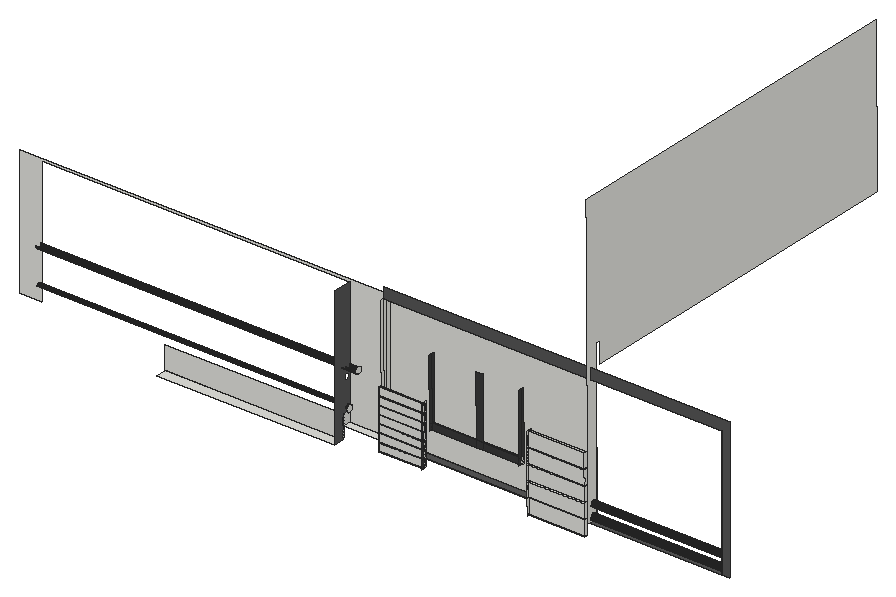
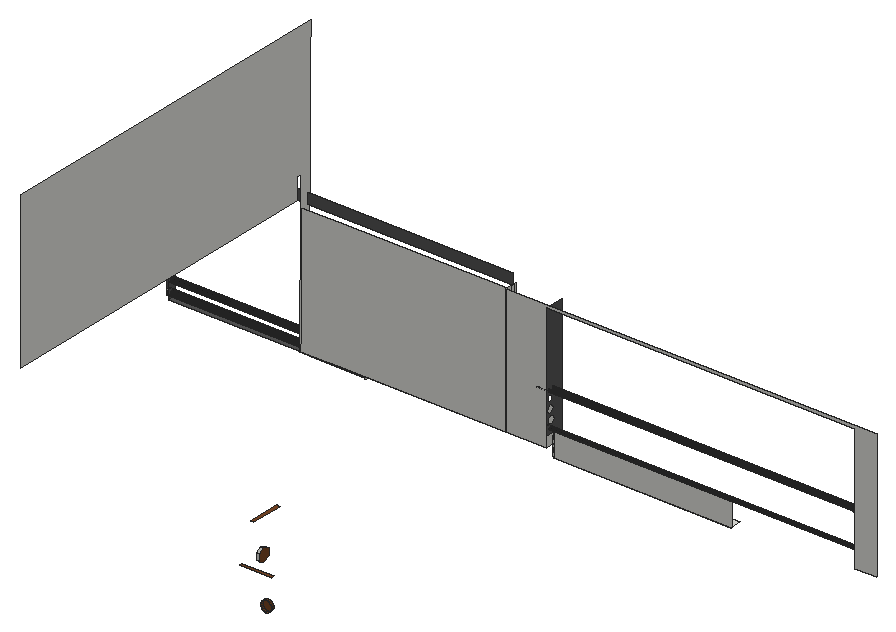
# SketchUp Ruby script. Lengths in inches.
U = 1.inch
M = Sketchup.active_model
def pt(a) = Geom::Point3d.new(a.map { |v| v * U })
def face(e, loops, mat)
  f = e.add_face(loops[0].map { |a| pt(a) })
  loops[1..].each { |l| e.add_face(l.map { |a| pt(a) }).erase! }
  f.material = f.back_material = mat if mat
  f
end
# faces: each face lists its corners as indices into pts; further lists are holes
def faces(e, pts, list, mat = nil) = list.each { |f| face(e, (f[0].is_a?(Array) ? f : [f]).map { |l| l.map { |i| pts[i] } }, mat) }
# xy, xz, yz: faces in a plane at the given z, y or x. An outline is a flat list of corners, or four numbers for a rectangle; further outlines are holes
def ring(l) = l.size == 4 ? [[l[0], l[1]], [l[2], l[1]], [l[2], l[3]], [l[0], l[3]]] : l.each_slice(2).to_a
def flat(e, list, mat, &to3) = list.each { |f| face(e, (f[0].is_a?(Array) ? f : [f]).map { |l| ring(l).map { |u, v| to3.(u, v) } }, mat) }
def xy(e, z, list, mat = nil) = flat(e, list, mat) { |x, y| [x, y, z] }
def xz(e, y, list, mat = nil) = flat(e, list, mat) { |x, z| [x, y, z] }
def yz(e, x, list, mat = nil) = flat(e, list, mat) { |y, z| [x, y, z] }
def lines(e, pts, list) = list.each { |a, b| e.add_line(pt(pts[a]), pt(pts[b])) }
# prism: a flat outline (further loops are holes) pulled along v
def prism(e, loops, v, mat = nil)
  f = face(e, loops, mat); d = Geom::Vector3d.new(v.map { |x| x * U })
  f.pushpull(f.normal.samedirection?(d) ? d.length : -d.length)
end
def box(e, o, s, mat = nil) = prism(e, [[o, [o[0] + s[0], o[1], o[2]], [o[0] + s[0], o[1] + s[1], o[2]], [o[0], o[1] + s[1], o[2]]]], [0, 0, s[2]], mat)
def at(x, y, z, deg = 0) = Geom::Transformation.translation(pt([x, y, z])) * Geom::Transformation.rotation(ORIGIN, Z_AXIS, deg.degrees)
def axes(o, x, y, z) = Geom::Transformation.new([*x, 0, *y, 0, *z, 0, *pt(o).to_a, 1])
def part(name) = M.definitions.add(name)
# library, detail: a bought-in or finely detailed component or shape, given as its bounding box
def library(name, o, s) = part(name).tap { |d| box(d.entities, o, s) }
def detail(e, o, s) = box(e.add_group.entities, o, s)
def put(e, d, t, mat = nil) = e.add_instance(d, t).tap { |i| i.material = mat if mat }
def group(e, t, mat = nil) = e.add_group.tap { |g| g.transformation = t; g.material = mat if mat }.entities
root = M.entities
M.materials.add("[0136_Charcoal]").color = [35, 35, 35]
M.materials.add("[Color M06]").color = [86, 86, 86]
M.materials.add("[Color M07]").color = [58, 58, 58]
M.materials.add("[Wood Veneer 01]").color = [120, 70, 37]
xy(root,214.25,[[350.625,15,549.5625,26.8125]])
xy(root,228,[[549.5625,27,595.0625,36]])
xy(root,228,[[595.0625,27,973.625,36]],"[Color M06]")
xy(root,276,[[614,330.04,617,366.04],[539.92,430.1875,575.92,433.1875]],"[Wood Veneer 01]")
xy(root,286.06,[[762.91,22.06,825.84,22.1875]])
xz(root,26.8125,[[349.93,214.25,549.5625,240]])
xz(root,27,[[595.0625,227.94,784.34,228],[595.0625,227.94,825.84,228],[784.34,227.94,825.84,228]])
xz(root,27,[[973.625,228,982.625,228,982.625,384,595.0625,384,595.0625,372,973.625,372]],"[Color M06]")
xz(root,36,[[180.5,228,180.5,372,595.0625,372,595.0625,228,549.5625,228,549.5625,368.875,204.375,368.875,204.375,228]])
xz(root,348.94,[[611,235.8,614,243.23]],"[Wood Veneer 01]")
xz(root,361.82,[[611,235.8,614,243.23]])
xz(root,427.1875,[[548.71,236.42,550.32,236.63,551.81,237.25,553.09,238.24,554.07,239.52,554.69,241.01,554.9,242.61,554.69,244.21,554.07,245.7,553.09,246.99,551.81,247.97,550.32,248.59,548.71,248.8,547.11,248.59,545.62,247.97,544.34,246.99,543.36,245.7,542.74,244.21,542.53,242.61,542.74,241.01,543.36,239.52,544.34,238.24,545.62,237.25,547.11,236.63]],"[Wood Veneer 01]")
yz(root,548.3125,[[31.79,251.75,32.66,251.86,33.47,252.2,34.17,252.73,34.71,253.43,35.05,254.25,35.16,255.12,35.05,255.99,34.71,256.81,34.17,257.51,33.47,258.04,32.66,258.38,31.79,258.5,30.91,258.38,30.1,258.04,29.4,257.51,28.86,256.81,28.53,255.99,28.41,255.12,28.53,254.25,28.86,253.43,29.4,252.73,30.1,252.2,30.91,251.86]])
yz(root,549.4375,[[31.79,262.25,32.66,262.36,33.47,262.7,34.17,263.23,34.71,263.93,35.05,264.75,35.16,265.62,35.05,266.49,34.71,267.31,34.17,268.01,33.47,268.54,32.66,268.88,31.79,269,30.91,268.88,30.1,268.54,29.4,268.01,28.86,267.31,28.53,266.49,28.41,265.62,28.53,264.75,28.86,263.93,29.4,263.23,30.1,262.7,30.91,262.36]])
yz(root,549.5625,[[26.8125,216.1875,27,228],[26.8125,228,27,240],[27,228,36,240]])
yz(root,549.5625,[[[15,214.25,15,368.875,36,368.875,36,240,26.8125,240,26.8125,214.25],[31.79,272.75,32.66,272.86,33.47,273.2,34.17,273.73,34.71,274.43,35.05,275.25,35.16,276.12,35.05,276.99,34.71,277.81,34.17,278.51,33.47,279.04,32.66,279.38,31.79,279.5,30.91,279.38,30.1,279.04,29.4,278.51,28.86,277.81,28.53,276.99,28.41,276.12,28.53,275.25,28.86,274.43,29.4,273.73,30.1,273.2,30.91,272.86]]],"[Color M06]")
yz(root,552.875,[[31.79,241.25,32.66,241.36,33.47,241.7,34.17,242.23,34.71,242.93,35.05,243.75,35.16,244.62,35.05,245.49,34.71,246.31,34.17,247.01,33.47,247.54,32.66,247.88,31.79,248,30.91,247.88,30.1,247.54,29.4,247.01,28.86,246.31,28.53,245.49,28.41,244.62,28.53,243.75,28.86,242.93,29.4,242.23,30.1,241.7,30.91,241.36]])
yz(root,562.875,[[31.79,283.25,32.66,283.36,33.47,283.7,34.17,284.23,34.71,284.93,35.05,285.75,35.16,286.62,35.05,287.49,34.71,288.31,34.17,289.01,33.47,289.54,32.66,289.88,31.79,290,30.91,289.88,30.1,289.54,29.4,289.01,28.86,288.31,28.53,287.49,28.41,286.62,28.53,285.75,28.86,284.93,29.4,284.23,30.1,283.7,30.91,283.36]])
yz(root,595.0625,[[20.53,222.36,20.47,230.59,22.09,230.6,22.14,222.37],[27,227.94,27,227.98,30,228,30,227.96],[30,227.96,30,228,36,228],[24,227.98,27,228,26.0625,371.94,23.0625,371.92],[27,227.98,27,228,30,228],
  [27,228,30,228,29.0625,371.96,26.0625,371.94],[30,228,36,228,35.0625,372,29.0625,371.96],[36,228,36,372,35.0625,372],[20.47,231.55,20.41,239.78,22.09,239.79,22.14,231.56],[20.41,240.74,20.35,248.96,22.09,248.97,22.14,240.75],
  [20.35,249.92,20.29,258.15,22.09,258.16,22.14,249.93],[20.29,259.11,20.23,267.34,22.09,267.35,22.14,259.12],[20.23,268.3,20.17,276.52,22.09,276.54,22.14,268.31],[20.16,278.11,20.11,286.34,22.09,286.35,22.14,278.12]])
yz(root,611,[[355.38,232.08,348.94,235.8,348.94,243.23,355.38,246.95,361.82,243.23,361.82,235.8]],"[Wood Veneer 01]")
yz(root,644.47,[[21.04,221.4,21.04,222.36,22.14,222.37,24.04,222.38,24.04,221.42,22.09,221.41],[20.53,222.36,20.47,230.59,20.98,230.59,21.04,222.36],[21.04,222.36,20.98,230.59,22.09,230.6,22.14,222.37],[22.14,222.37,22.09,230.6,23.98,230.61,24.04,222.38],[20.98,230.59,20.98,231.55,22.14,231.56,23.98,231.57,23.98,230.61,22.09,230.6],
  [20.47,231.55,20.41,239.78,20.92,239.78,20.98,231.55],[20.98,231.55,20.92,239.78,22.09,239.79,22.14,231.56],[22.14,231.56,22.09,239.79,23.92,239.8,23.98,231.57],[20.92,239.78,20.92,240.74,22.14,240.75,23.92,240.76,23.92,239.8,22.09,239.79],[20.41,240.74,20.35,248.96,20.86,248.97,20.92,240.74],
  [20.92,240.74,20.86,248.97,22.09,248.97,22.14,240.75],[22.14,240.75,22.09,248.97,23.86,248.99,23.92,240.76],[20.86,248.97,20.86,249.93,22.14,249.93,23.86,249.95,23.86,248.99,22.09,248.97],[20.35,249.92,20.29,258.15,20.8,258.15,20.86,249.93],[20.86,249.93,20.8,258.15,22.09,258.16,22.14,249.93],
  [22.14,249.93,22.09,258.16,23.8,258.17,23.86,249.95],[20.8,258.15,20.8,259.11,22.14,259.12,23.8,259.13,23.8,258.17,22.09,258.16],[20.29,259.11,20.23,267.34,20.74,267.34,20.8,259.11],[20.8,259.11,20.74,267.34,22.09,267.35,22.14,259.12],[22.14,259.12,22.09,267.35,23.74,267.36,23.8,259.13],
  [20.74,267.34,20.74,268.3,22.14,268.31,23.74,268.32,23.74,267.36,22.09,267.35],[20.23,268.3,20.17,276.52,20.68,276.53,20.74,268.3],[20.74,268.3,20.68,276.53,22.09,276.54,22.14,268.31],[22.14,268.31,22.09,276.54,23.68,276.55,23.74,268.32],[20.68,276.53,20.67,278.11,22.14,278.12,23.67,278.13,23.68,276.55,22.09,276.54],
  [20.16,278.11,20.11,286.34,20.62,286.34,20.67,278.11],[20.67,278.11,20.62,286.34,22.09,286.35,22.14,278.12],[22.14,278.12,22.09,286.35,23.62,286.36,23.67,278.13],[20.62,286.34,20.61,287.92,22.14,287.93,23.61,287.94,23.62,286.36,22.09,286.35]])
yz(root,644.47,[[18.04,221.39,18.04,222.34,20.53,222.36,21.04,222.36,21.04,221.4,20.53,221.4],[18.04,222.34,17.98,230.57,20.47,230.59,20.53,222.36],[17.98,230.57,17.98,231.53,20.47,231.55,20.98,231.55,20.98,230.59,20.47,230.59],[17.98,231.53,17.92,239.76,20.41,239.78,20.47,231.55],[17.92,239.76,17.92,240.72,20.41,240.74,20.92,240.74,20.92,239.78,20.41,239.78],
  [17.92,240.72,17.86,248.95,20.35,248.96,20.41,240.74],[17.86,248.95,17.86,249.91,20.35,249.92,20.86,249.93,20.86,248.97,20.35,248.96],[17.86,249.91,17.8,258.13,20.29,258.15,20.35,249.92],[17.8,258.13,17.8,259.09,20.29,259.11,20.8,259.11,20.8,258.15,20.29,258.15],[17.8,259.09,17.74,267.32,20.23,267.34,20.29,259.11],
  [17.74,267.32,17.74,268.28,20.23,268.3,20.74,268.3,20.74,267.34,20.23,267.34],[17.74,268.28,17.68,276.51,20.17,276.52,20.23,268.3],[17.68,276.51,17.67,278.09,20.16,278.11,20.67,278.11,20.68,276.53,20.17,276.52],[17.67,278.09,17.62,286.32,20.11,286.34,20.16,278.11],[17.62,286.32,17.61,287.9,20.1,287.92,20.61,287.92,20.62,286.34,20.11,286.34]],"[Color M07]")
yz(root,653.47,[[20.77,263.62,22.78,263.63,22.73,270.75,20.72,270.73],[22.78,263.63,23.77,263.64,23.72,270.75,22.73,270.75]])
yz(root,653.47,[[17.77,263.6,20.77,263.62,20.72,270.73,17.72,270.71],[17.72,270.71,20.72,270.73,20.27,339.74,17.27,339.72],[20.72,270.73,22.73,270.75,23.72,270.75,23.27,339.76,22.78,339.76,20.27,339.74]],"[Color M07]")
yz(root,753.91,[[20.77,263.62,20.72,270.73,22.73,270.75,22.78,263.63],[22.78,263.63,22.73,270.75,23.72,270.75,23.77,263.64]])
yz(root,753.91,[[17.77,263.6,17.72,270.71,20.72,270.73,20.77,263.62],[17.72,270.71,17.27,339.72,20.27,339.74,20.72,270.73],[20.72,270.73,20.27,339.74,22.78,339.76,23.27,339.76,23.72,270.75,22.73,270.75]],"[Color M07]")
yz(root,762.91,[[18.07,216.95,19.51,216.96,21.07,216.97,21.0625,218.3,19.5,218.29,18.0625,218.28],[21.07,216.97,21.0625,218.3,22.1875,218.31,24.0625,218.32,24.07,216.99,22.09,216.97],[18.0625,218.28,19.5,218.29,19.4,233.89,17.96,233.88],[19.5,218.29,21.0625,218.3,20.96,233.9,19.4,233.89],[21.0625,218.3,22.1875,218.31,22.09,233.91,20.96,233.9],
  [22.1875,218.31,22.09,233.91,23.96,233.92,24.0625,218.32],[17.96,233.88,19.4,233.89,20.96,233.9,20.95,235.24,19.39,235.23,17.95,235.22],[20.96,233.9,20.95,235.24,22.1875,235.25,23.95,235.26,23.96,233.92,22.09,233.91],[17.95,235.22,19.39,235.23,19.29,250.83,17.85,250.82],[19.39,235.23,20.95,235.24,20.85,250.84,19.29,250.83],
  [20.95,235.24,22.1875,235.25,22.09,250.85,20.85,250.84],[22.1875,235.25,22.09,250.85,23.85,250.86,23.95,235.26],[17.85,250.82,19.29,250.83,20.85,250.84,20.84,252.18,19.28,252.17,17.84,252.16],[20.85,250.84,20.84,252.18,22.1875,252.19,23.84,252.2,23.85,250.86,22.09,250.85],[17.84,252.16,19.28,252.17,19.18,267.77,17.74,267.76],
  [19.28,252.17,20.84,252.18,20.74,267.78,19.18,267.77],[20.84,252.18,22.1875,252.19,22.09,267.79,20.74,267.78],[22.1875,252.19,22.09,267.79,23.74,267.8,23.84,252.2],[17.74,267.76,19.18,267.77,20.74,267.78,20.73,269.11,19.17,269.1,17.73,269.09],[20.74,267.78,20.73,269.11,22.1875,269.12,23.73,269.13,23.74,267.8,22.09,267.79],
  [17.73,269.09,19.17,269.1,19.07,284.7,17.63,284.7],[19.17,269.1,20.73,269.11,20.63,284.71,19.07,284.7],[20.73,269.11,22.1875,269.12,22.09,284.72,20.63,284.71],[22.1875,269.12,22.09,284.72,23.63,284.73,23.73,269.13],[17.63,284.7,19.07,284.7,20.63,284.71,20.62,286.05,19.06,286.04,17.62,286.03],
  [20.63,284.71,20.62,286.05,22.06,286.06,22.1875,286.06,23.62,286.07,23.63,284.73,22.09,284.72],[17.62,286.03,19.06,286.04,18.96,301.64,17.52,301.63],[19.06,286.04,20.62,286.05,20.52,301.65,18.96,301.64],[20.62,286.05,22.06,286.06,21.96,301.66,20.52,301.65],[22.06,286.06,22.1875,286.06,22.09,301.66,21.96,301.66],
  [22.1875,286.06,22.09,301.66,23.52,301.67,23.62,286.07]])
yz(root,825.84,[[19.5,218.29,22.1875,218.31,22.09,233.91,19.4,233.89],[[27,227.94,36,228,35.0625,372,34.85,405.125,40.66,405.16,40.8125,381.35,428.06,383.87,426.93,557.18,21.875,554.54,21.89,551.83,22.09,521.85,22.1875,506.25,24,227.98,27,228],[31.09,243.06,30.27,243.17,29.5,243.49,28.84,244,28.33,244.66,28.02,245.43,27.91,246.25,28.02,247.08,28.33,247.85,28.84,248.51,29.5,249.01,30.27,249.33,31.09,249.44,31.92,249.33,32.6875,249.01,33.35,248.51,33.85,247.85,34.17,247.08,34.28,246.25,34.17,245.43,33.85,244.66,33.35,244,32.6875,243.49,31.92,243.17],[31.09,229.75,30.27,229.86,29.5,230.18,28.84,230.6875,28.33,231.35,28.02,232.11,27.91,232.94,28.02,233.76,28.33,234.53,28.84,235.19,29.5,235.7,30.27,236.02,31.09,236.13,31.92,236.02,32.6875,235.7,33.35,235.19,33.85,234.53,34.17,233.76,34.28,232.94,34.17,232.11,33.85,231.35,33.35,230.6875,32.6875,230.18,31.92,229.86]],[31.09,229.75,30.27,229.86,29.5,230.18,28.84,230.6875,28.33,231.35,28.02,232.11,27.91,232.94,28.02,233.76,28.33,234.53,28.84,235.19,29.5,235.7,30.27,236.02,31.09,236.13,31.92,236.02,32.6875,235.7,33.35,235.19,33.85,234.53,34.17,233.76,34.28,232.94,34.17,232.11,33.85,231.35,33.35,230.6875,32.6875,230.18,31.92,229.86],[19.39,235.23,22.1875,235.25,22.09,250.85,19.29,250.83],[31.09,243.06,30.27,243.17,29.5,243.49,28.84,244,28.33,244.66,28.02,245.43,27.91,246.25,28.02,247.08,28.33,247.85,28.84,248.51,29.5,249.01,30.27,249.33,31.09,249.44,31.92,249.33,32.6875,249.01,33.35,248.51,33.85,247.85,34.17,247.08,34.28,246.25,34.17,245.43,33.85,244.66,33.35,244,32.6875,243.49,31.92,243.17],
  [19.28,252.17,22.1875,252.19,22.09,267.79,19.18,267.77],[19.17,269.1,22.1875,269.12,22.09,284.72,19.07,284.7],[19.06,286.04,22.06,286.06,21.96,301.66,18.96,301.64],[22.06,286.06,22.1875,286.06,22.09,301.66,21.96,301.66]])
yz(root,973.625,[[27,228,35.0625,372]],"[Color M06]")
yz(root,975.03,[[31.09,243.06,31.92,243.17,32.6875,243.49,33.35,244,33.85,244.66,34.17,245.43,34.28,246.25,34.17,247.08,33.85,247.85,33.35,248.51,32.6875,249.01,31.92,249.33,31.09,249.44,30.27,249.33,29.5,249.01,28.84,248.51,28.33,247.85,28.02,247.08,27.91,246.25,28.02,245.43,28.33,244.66,28.84,244,29.5,243.49,30.27,243.17]])
yz(root,977.16,[[31.09,229.75,31.92,229.86,32.6875,230.18,33.35,230.6875,33.85,231.35,34.17,232.11,34.28,232.94,34.17,233.76,33.85,234.53,33.35,235.19,32.6875,235.7,31.92,236.02,31.09,236.13,30.27,236.02,29.5,235.7,28.84,235.19,28.33,234.53,28.02,233.76,27.91,232.94,28.02,232.11,28.33,231.35,28.84,230.6875,29.5,230.18,30.27,229.86]])
p = [[825.84,22.09,216.97],[762.91,22.09,216.97],[762.91,21.07,216.97],[762.91,19.51,216.96],[825.84,19.51,216.96],[762.91,19.4,233.89],
  [762.91,19.5,218.29],[825.84,19.5,218.29],[825.84,19.4,233.89],[762.91,22.1875,218.31],[825.84,22.1875,218.31],[762.91,21.0625,218.3],
  [762.91,22.09,233.91],[825.84,22.09,233.91],[644.47,22.09,221.41],[595.0625,22.09,221.41],[595.0625,20.53,221.4],[644.47,20.53,221.4],
  [644.47,21.04,221.4],[595.0625,20.47,230.59],[595.0625,20.53,222.36],[644.47,20.53,222.36],[644.47,20.47,230.59],[595.0625,22.14,222.37],
  [644.47,22.14,222.37],[644.47,21.04,222.36],[595.0625,22.09,230.6],[644.47,22.09,230.6],[595.0625,30,227.96],[825.84,30,227.96],
  [825.84,27,227.94],[784.34,27,227.94],[595.0625,27,227.94],[595.0625,36,228],[784.34,36,228],[825.84,36,228],
  [595.0625,35.0625,372],[784.34,35.0625,372],[825.84,35.0625,372],[825.84,30.27,229.86],[825.84,31.09,229.75],[977.16,31.09,229.75],
  [977.16,30.27,229.86],[825.84,31.92,229.86],[977.16,31.92,229.86],[825.84,29.5,230.18],[977.16,29.5,230.18],[825.84,32.6875,230.18],
  [977.16,32.6875,230.18],[825.84,28.84,230.6875],[977.16,28.84,230.6875],[825.84,33.35,230.6875],[977.16,33.35,230.6875],[644.47,20.98,230.59],
  [825.84,28.33,231.35],[977.16,28.33,231.35],[825.84,33.85,231.35],[977.16,33.85,231.35],[825.84,28.02,232.11],[977.16,28.02,232.11],
  [825.84,34.17,232.11],[977.16,34.17,232.11],[595.0625,20.41,239.78],[595.0625,20.47,231.55],[644.47,20.47,231.55],[644.47,20.41,239.78],
  [595.0625,22.14,231.56],[644.47,22.14,231.56],[644.47,20.98,231.55],[595.0625,22.09,239.79],[644.47,22.09,239.79],[825.84,27.91,232.94],
  [977.16,27.91,232.94],[825.84,34.28,232.94],[977.16,34.28,232.94],[614,355.38,232.08],[614,348.94,235.8],[611,348.94,235.8],
  [611,355.38,232.08],[614,361.82,235.8],[611,361.82,235.8],[825.84,28.02,233.76],[977.16,28.02,233.76],[825.84,34.17,233.76],
  [977.16,34.17,233.76],[825.84,28.33,234.53],[977.16,28.33,234.53],[825.84,33.85,234.53],[977.16,33.85,234.53],[762.91,20.96,233.9],
  [825.84,28.84,235.19],[977.16,28.84,235.19],[825.84,33.35,235.19],[977.16,33.35,235.19],[762.91,19.29,250.83],[762.91,19.39,235.23],
  [825.84,19.39,235.23],[825.84,19.29,250.83],[762.91,22.1875,235.25],[825.84,22.1875,235.25],[762.91,20.95,235.24],[762.91,22.09,250.85],
  [825.84,22.09,250.85],[825.84,29.5,235.7],[977.16,29.5,235.7],[825.84,32.6875,235.7],[977.16,32.6875,235.7],[825.84,30.27,236.02],
  [977.16,30.27,236.02],[825.84,31.92,236.02],[977.16,31.92,236.02],[825.84,31.09,236.13],[977.16,31.09,236.13],[547.11,430.1875,236.63],
  [548.71,430.1875,236.42],[548.71,427.1875,236.42],[547.11,427.1875,236.63],[550.32,430.1875,236.63],[550.32,427.1875,236.63],[545.62,430.1875,237.25],
  [545.62,427.1875,237.25],[551.81,430.1875,237.25],[551.81,427.1875,237.25],[544.34,430.1875,238.24],[544.34,427.1875,238.24],[553.09,430.1875,238.24],
  [553.09,427.1875,238.24],[543.36,430.1875,239.52],[543.36,427.1875,239.52],[554.07,430.1875,239.52],[554.07,427.1875,239.52],[542.74,430.1875,241.01],
  [542.74,427.1875,241.01],[554.69,430.1875,241.01],[554.69,427.1875,241.01],[644.47,20.92,239.78],[595.0625,20.35,248.96],[595.0625,20.41,240.74],
  [644.47,20.41,240.74],[644.47,20.35,248.96],[595.0625,22.14,240.75],[644.47,22.14,240.75],[644.47,20.92,240.74],[595.0625,22.09,248.97],
  [644.47,22.09,248.97],[542.53,430.1875,242.61],[542.53,427.1875,242.61],[554.9,430.1875,242.61],[554.9,427.1875,242.61],[542.74,430.1875,244.21],
  [542.74,427.1875,244.21],[554.69,430.1875,244.21],[554.69,427.1875,244.21],[825.84,30.27,243.17],[825.84,31.09,243.06],[975.03,31.09,243.06],
  [975.03,30.27,243.17],[825.84,31.92,243.17],[975.03,31.92,243.17],[825.84,29.5,243.49],[975.03,29.5,243.49],[825.84,32.6875,243.49],
  [975.03,32.6875,243.49],[614,348.94,243.23],[614,355.38,246.95],[611,355.38,246.95],[611,348.94,243.23],[614,361.82,243.23],
  [611,361.82,243.23],[825.84,28.84,244],[975.03,28.84,244],[825.84,33.35,244],[975.03,33.35,244],[825.84,28.33,244.66],
  [975.03,28.33,244.66],[825.84,33.85,244.66],[975.03,33.85,244.66],[543.36,430.1875,245.7],[543.36,427.1875,245.7],[554.07,430.1875,245.7],
  [554.07,427.1875,245.7],[825.84,28.02,245.43],[975.03,28.02,245.43],[825.84,34.17,245.43],[975.03,34.17,245.43],[825.84,27.91,246.25],
  [975.03,27.91,246.25],[825.84,34.28,246.25],[975.03,34.28,246.25],[544.34,430.1875,246.99],[544.34,427.1875,246.99],[553.09,430.1875,246.99],
  [553.09,427.1875,246.99],[825.84,28.02,247.08],[975.03,28.02,247.08],[204.375,29.4,247.01],[204.375,28.86,246.31],[552.875,28.86,246.31],
  [552.875,29.4,247.01],[204.375,34.71,246.31],[204.375,34.17,247.01],[552.875,34.17,247.01],[552.875,34.71,246.31],[825.84,34.17,247.08],
  [975.03,34.17,247.08],[204.375,30.1,247.54],[552.875,30.1,247.54],[204.375,33.47,247.54],[552.875,33.47,247.54],[545.62,430.1875,247.97],
  [545.62,427.1875,247.97],[551.81,430.1875,247.97],[551.81,427.1875,247.97],[825.84,28.33,247.85],[975.03,28.33,247.85],[825.84,33.85,247.85],
  [975.03,33.85,247.85],[204.375,30.91,247.88],[552.875,30.91,247.88],[204.375,32.66,247.88],[552.875,32.66,247.88],[825.84,28.84,248.51],
  [975.03,28.84,248.51],[825.84,33.35,248.51],[975.03,33.35,248.51],[204.375,31.79,248],[552.875,31.79,248],[547.11,430.1875,248.59],
  [547.11,427.1875,248.59],[550.32,430.1875,248.59],[550.32,427.1875,248.59],[825.84,29.5,249.01],[975.03,29.5,249.01],[825.84,32.6875,249.01],
  [975.03,32.6875,249.01],[548.71,430.1875,248.8],[548.71,427.1875,248.8],[644.47,20.86,248.97],[825.84,30.27,249.33],[975.03,30.27,249.33],
  [825.84,31.92,249.33],[975.03,31.92,249.33],[825.84,31.09,249.44],[975.03,31.09,249.44],[595.0625,20.29,258.15],[595.0625,20.35,249.92],
  [644.47,20.35,249.92],[644.47,20.29,258.15],[595.0625,22.14,249.93],[644.47,22.14,249.93],[644.47,20.86,249.93],[595.0625,22.09,258.16],
  [644.47,22.09,258.16],[762.91,20.85,250.84],[762.91,19.18,267.77],[762.91,19.28,252.17],[825.84,19.28,252.17],[825.84,19.18,267.77],
  [762.91,22.1875,252.19],[825.84,22.1875,252.19],[762.91,20.84,252.18],[762.91,22.09,267.79],[825.84,22.09,267.79],[644.47,20.8,258.15],
  [595.0625,20.23,267.34],[595.0625,20.29,259.11],[644.47,20.29,259.11],[644.47,20.23,267.34],[595.0625,22.14,259.12],[644.47,22.14,259.12],
  [644.47,20.8,259.11],[595.0625,22.09,267.35],[644.47,22.09,267.35],[653.47,20.77,263.62],[703.69,20.77,263.62],[703.69,20.72,270.73],
  [653.47,20.72,270.73],[710.84,20.72,270.73],[710.84,20.77,263.62],[753.91,20.72,270.73],[753.91,20.77,263.62],[653.47,22.78,263.63],
  [703.69,22.78,263.63],[710.84,22.78,263.63],[753.91,22.78,263.63],[653.47,22.73,270.75],[703.69,22.73,270.75],[710.84,22.73,270.75],
  [753.91,22.73,270.75],[644.47,20.74,267.34],[762.91,20.74,267.78],[595.0625,20.17,276.52],[595.0625,20.23,268.3],[644.47,20.23,268.3],
  [644.47,20.17,276.52],[595.0625,22.14,268.31],[644.47,22.14,268.31],[644.47,20.74,268.3],[595.0625,22.09,276.54],[644.47,22.09,276.54],
  [762.91,19.07,284.7],[762.91,19.17,269.1],[825.84,19.17,269.1],[825.84,19.07,284.7],[762.91,22.1875,269.12],[825.84,22.1875,269.12],
  [762.91,20.73,269.11],[762.91,22.09,284.72],[825.84,22.09,284.72],[710.84,20.27,339.74],[703.69,20.27,339.74],[644.47,20.68,276.53],
  [595.0625,20.11,286.34],[595.0625,20.16,278.11],[644.47,20.16,278.11],[644.47,20.11,286.34],[595.0625,22.14,278.12],[644.47,22.14,278.12],
  [644.47,20.67,278.11],[595.0625,22.09,286.35],[644.47,22.09,286.35],[204.375,30.91,283.36],[204.375,31.79,283.25],[562.875,31.79,283.25],
  [562.875,30.91,283.36],[204.375,32.66,283.36],[562.875,32.66,283.36],[204.375,30.1,283.7],[562.875,30.1,283.7],[204.375,33.47,283.7],
  [562.875,33.47,283.7],[204.375,29.4,284.23],[562.875,29.4,284.23],[204.375,34.17,284.23],[562.875,34.17,284.23],[204.375,28.86,284.93],
  [562.875,28.86,284.93],[204.375,34.71,284.93],[562.875,34.71,284.93],[762.91,20.63,284.71],[204.375,28.53,285.75],[562.875,28.53,285.75],
  [204.375,35.05,285.75],[562.875,35.05,285.75],[204.375,28.41,286.62],[562.875,28.41,286.62],[204.375,35.16,286.62],[562.875,35.16,286.62],
  [762.91,18.96,301.64],[762.91,19.06,286.04],[825.84,19.06,286.04],[825.84,18.96,301.64],[762.91,22.06,286.06],[825.84,22.06,286.06],
  [762.91,20.62,286.05],[762.91,21.96,301.66],[825.84,21.96,301.66],[762.91,22.1875,286.06],[762.91,22.09,301.66],[825.84,22.09,301.66],
  [825.84,22.1875,286.06],[644.47,20.62,286.34],[204.375,28.53,287.49],[562.875,28.53,287.49],[204.375,35.05,287.49],[562.875,35.05,287.49],
  [784.34,27,228],[784.34,24,227.98]]
faces(root,p,[[0,1,2,3,4],[5,6,7,8],[9,10,7,6,11],[9,12,13,10],[14,15,16,17,18],[19,20,21,22],[23,24,25,21,20],[23,26,27,24],
  [28,29,30,31,32],[33,34,35,29,28],[33,36,37,38,35,34],[27,26,19,22,53],[62,63,64,65],[66,67,68,64,63],[66,69,70,67],[79,75,78,80],
  [13,12,89,5,8],[94,95,96,97],[98,99,96,95,100],[98,101,102,99],[70,69,62,65,135],[136,137,138,139],[140,141,142,138,137],[140,143,144,141],
  [164,167,168,165],[144,143,136,139,237],[244,245,246,247],[248,249,250,246,245],[248,251,252,249],[102,101,253,94,97],[254,255,256,257],[258,259,256,255,260],
  [258,261,262,259],[252,251,244,247,263],[264,265,266,267],[268,269,270,266,265],[268,271,272,269],[282,283,278,274],[282,281,285,286,287,288,284,283],[272,271,264,267,289],
  [262,261,290,254,257],[291,292,293,294],[295,296,297,293,292],[295,298,299,296],[300,301,302,303],[304,305,302,301,306],[304,307,308,305],[286,285,276,275],
  [287,286,275,277],[288,287,277,279],[299,298,291,294,311],[312,313,314,315],[316,317,318,314,313],[316,319,320,317],[308,307,339,300,303],[348,349,350,351],
  [352,353,350,349,354],[352,355,356,353],[357,358,359,360],[320,319,312,315,361]])
faces(root,p,[[39,40,41,42],[40,43,44,41],[45,39,42,46],[43,47,48,44],[49,45,46,50],[47,51,52,48],[54,49,50,55],[51,56,57,52],
  [58,54,55,59],[56,60,61,57],[71,58,59,72],[60,73,74,61],[81,71,72,82],[73,83,84,74],[85,81,82,86],[83,87,88,84],
  [90,85,86,91],[87,92,93,88],[103,90,91,104],[92,105,106,93],[107,103,104,108],[105,109,110,106],[111,107,108,112],[109,111,112,110],
  [153,154,155,156],[154,157,158,155],[159,153,156,160],[157,161,162,158],[169,159,160,170],[161,171,172,162],[173,169,170,174],[171,175,176,172],
  [181,173,174,182],[175,183,184,176],[185,181,182,186],[183,187,188,184],[193,185,186,194],[195,196,197,198],[199,200,201,202],[187,203,204,188],
  [205,195,198,206],[200,207,208,201],[213,193,194,214],[203,215,216,204],[217,205,206,218],[207,219,220,208],[221,213,214,222],[215,223,224,216],
  [225,217,218,226],[219,225,226,220],[231,221,222,232],[223,233,234,224],[238,231,232,239],[233,240,241,234],[242,238,239,243],[240,242,243,241],
  [321,322,323,324],[322,325,326,323],[327,321,324,328],[325,329,330,326],[331,327,328,332],[329,333,334,330],[335,331,332,336],[333,337,338,334],
  [340,335,336,341],[337,342,343,338],[344,340,341,345],[342,346,347,343],[362,344,345,363],[346,364,365,347]],"[0136_Charcoal]")
faces(root,p,[[75,76,77,78],[113,114,115,116],[114,117,118,115],[119,113,116,120],[117,121,122,118],[123,119,120,124],[121,125,126,122],[127,123,124,128],
  [125,129,130,126],[131,127,128,132],[129,133,134,130],[145,131,132,146],[133,147,148,134],[149,145,146,150],[147,151,152,148],[163,164,165,166],
  [177,149,150,178],[151,179,180,152],[189,177,178,190],[179,191,192,180],[209,189,190,210],[191,211,212,192],[227,209,210,228],[211,229,230,212],
  [235,227,228,236],[229,235,236,230]],"[Wood Veneer 01]")
faces(root,p,[[273,274,275,276],[277,275,274,278],[279,277,278,280],[281,282,274,273],[283,284,280,278],[277,309,310,275]],"[Color M07]")
lines(root,p,[[366,367]])
